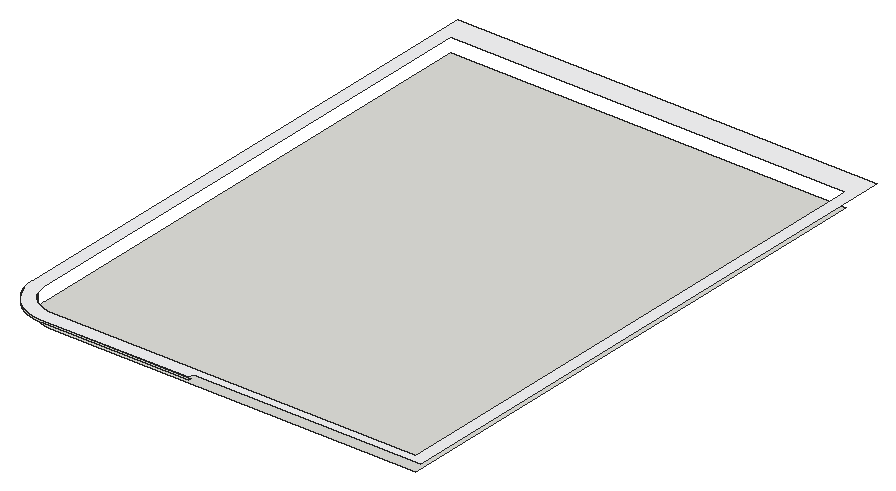
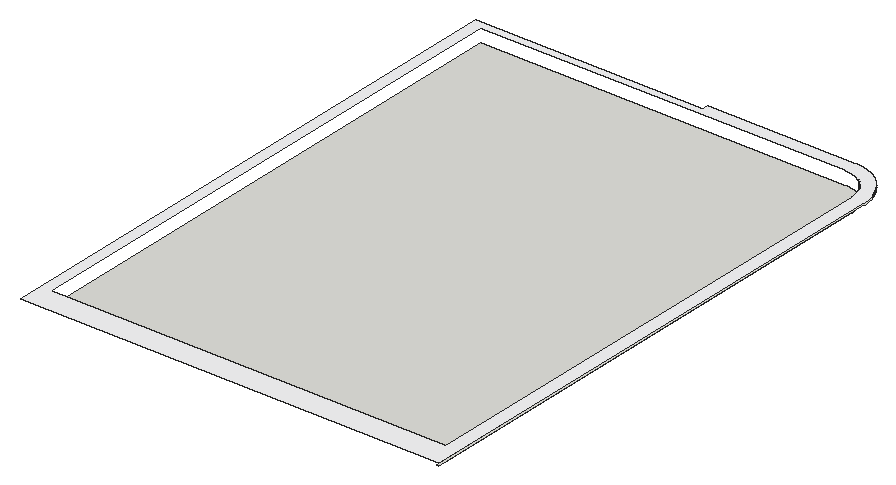
# SketchUp Ruby script. Lengths in inches.
U = 1.inch
M = Sketchup.active_model
def pt(a) = Geom::Point3d.new(a.map { |v| v * U })
def face(e, loops, mat)
  f = e.add_face(loops[0].map { |a| pt(a) })
  loops[1..].each { |l| e.add_face(l.map { |a| pt(a) }).erase! }
  f.material = f.back_material = mat if mat
  f
end
# faces: each face lists its corners as indices into pts; further lists are holes
def faces(e, pts, list, mat = nil) = list.each { |f| face(e, (f[0].is_a?(Array) ? f : [f]).map { |l| l.map { |i| pts[i] } }, mat) }
# xy, xz, yz: faces in a plane at the given z, y or x. An outline is a flat list of corners, or four numbers for a rectangle; further outlines are holes
def ring(l) = l.size == 4 ? [[l[0], l[1]], [l[2], l[1]], [l[2], l[3]], [l[0], l[3]]] : l.each_slice(2).to_a
def flat(e, list, mat, &to3) = list.each { |f| face(e, (f[0].is_a?(Array) ? f : [f]).map { |l| ring(l).map { |u, v| to3.(u, v) } }, mat) }
def xy(e, z, list, mat = nil) = flat(e, list, mat) { |x, y| [x, y, z] }
def xz(e, y, list, mat = nil) = flat(e, list, mat) { |x, z| [x, y, z] }
def yz(e, x, list, mat = nil) = flat(e, list, mat) { |y, z| [x, y, z] }
def lines(e, pts, list) = list.each { |a, b| e.add_line(pt(pts[a]), pt(pts[b])) }
# prism: a flat outline (further loops are holes) pulled along v
def prism(e, loops, v, mat = nil)
  f = face(e, loops, mat); d = Geom::Vector3d.new(v.map { |x| x * U })
  f.pushpull(f.normal.samedirection?(d) ? d.length : -d.length)
end
def box(e, o, s, mat = nil) = prism(e, [[o, [o[0] + s[0], o[1], o[2]], [o[0] + s[0], o[1] + s[1], o[2]], [o[0], o[1] + s[1], o[2]]]], [0, 0, s[2]], mat)
def at(x, y, z, deg = 0) = Geom::Transformation.translation(pt([x, y, z])) * Geom::Transformation.rotation(ORIGIN, Z_AXIS, deg.degrees)
def axes(o, x, y, z) = Geom::Transformation.new([*x, 0, *y, 0, *z, 0, *pt(o).to_a, 1])
def part(name) = M.definitions.add(name)
# library, detail: a bought-in or finely detailed component or shape, given as its bounding box
def library(name, o, s) = part(name).tap { |d| box(d.entities, o, s) }
def detail(e, o, s) = box(e.add_group.entities, o, s)
def put(e, d, t, mat = nil) = e.add_instance(d, t).tap { |i| i.material = mat if mat }
def group(e, t, mat = nil) = e.add_group.tap { |g| g.transformation = t; g.material = mat if mat }.entities
root = M.entities
M.materials.add("1122 AP 7994 PEACH ROSE").color = [254, 227, 201]
M.materials.add("[Quartz Light Grey]").color = [251, 251, 252]
xy(root,281.82,[[52.82,174,52.75,174.01,52.43,174.05,52.36,174.07,52.28,174.08,52.2,174.1,52.13,174.125,52.05,174.15,51.98,174.17,51.91,174.2,51.83,174.23,51.76,174.26,51.6875,174.29,51.62,174.33,51.55,174.36,51.41,174.44,51.35,174.48,51.28,174.53,51.22,174.57,51.15,174.62,50.97,174.77,50.86,174.88,50.8,174.93,50.6,175.17,50.55,175.24,50.51,175.3,50.46,175.37,50.42,175.43,50.34,175.57,50.31,175.64,50.27,175.71,50.18,175.92,50.15,176,50.13,176.07,50.1,176.15,50.08,176.22,50.0625,176.3,50.05,176.375,50.03,176.45,50.01,176.61,50,176.6875,49.99,176.76,49.99,176.84,49.98,176.92,49.98,177.08,49.99,177.16,49.99,177.24,50,177.3125,50.01,177.39,50.03,177.55,50.05,177.625,50.0625,177.7,50.08,177.78,50.1,177.85,50.13,177.93,50.15,178,50.18,178.08,50.27,178.29,50.31,178.36,50.34,178.43,50.42,178.57,50.46,178.63,50.51,178.7,50.55,178.76,50.6,178.83,50.8,179.07,50.86,179.12,50.97,179.23,51.15,179.38,51.22,179.43,51.28,179.47,51.35,179.52,51.41,179.56,51.55,179.64,51.62,179.67,51.6875,179.71,51.76,179.74,51.83,179.77,51.91,179.8,51.98,179.83,52.05,179.85,52.13,179.875,52.2,179.9,52.28,179.92,52.36,179.93,52.43,179.95,52.75,179.99,52.82,180,53.14,180,53.22,179.99,53.29,179.98,53.53,179.95,53.6,179.93,53.68,179.92,53.76,179.9,53.83,179.875,53.91,179.85,53.98,179.83,54.06,179.8,54.27,179.71,54.34,179.67,54.41,179.64,54.55,179.56,54.61,179.52,54.68,179.47,54.74,179.43,54.81,179.38,55.05,179.18,55.1,179.12,55.16,179.07,55.26,178.95,55.3125,178.89,55.36,178.83,55.41,178.76,55.45,178.7,55.5,178.63,55.54,178.57,55.62,178.43,55.65,178.36,55.6875,178.29,55.72,178.22,55.78,178.08,55.81,178,55.83,177.93,55.86,177.85,55.88,177.78,55.9,177.7,55.92,177.625,55.93,177.55,55.94,177.47,55.96,177.39,55.96,177.3125,55.97,177.24,55.98,177.16,55.98,176.84,55.97,176.76,55.96,176.6875,55.96,176.61,55.94,176.53,55.93,176.45,55.92,176.375,55.9,176.3,55.88,176.22,55.86,176.15,55.83,176.07,55.81,176,55.78,175.92,55.72,175.78,55.6875,175.71,55.65,175.64,55.62,175.57,55.54,175.43,55.5,175.37,55.45,175.3,55.41,175.24,55.36,175.17,55.3125,175.11,55.26,175.05,55.16,174.93,55.1,174.88,55.05,174.82,54.81,174.62,54.74,174.57,54.68,174.53,54.61,174.48,54.55,174.44,54.41,174.36,54.34,174.33,54.27,174.29,54.06,174.2,53.98,174.17,53.91,174.15,53.83,174.125,53.76,174.1,53.68,174.08,53.6,174.07,53.53,174.05,53.29,174.02,53.22,174.01,53.14,174],[164.84,174,164.76,174.01,164.6875,174.02,164.61,174.03,164.45,174.05,164.375,174.07,164.3,174.08,164.22,174.1,164.15,174.125,164.07,174.15,164,174.17,163.92,174.2,163.71,174.29,163.64,174.33,163.57,174.36,163.43,174.44,163.37,174.48,163.3,174.53,163.24,174.57,163.17,174.62,162.93,174.82,162.88,174.88,162.82,174.93,162.62,175.17,162.57,175.24,162.53,175.3,162.48,175.37,162.44,175.43,162.36,175.57,162.33,175.64,162.29,175.71,162.2,175.92,162.17,176,162.15,176.07,162.125,176.15,162.1,176.22,162.08,176.3,162.07,176.375,162.05,176.45,162.03,176.61,162.02,176.6875,162.01,176.76,162,176.84,162,177.16,162.01,177.24,162.02,177.3125,162.03,177.39,162.05,177.55,162.07,177.625,162.08,177.7,162.1,177.78,162.125,177.85,162.15,177.93,162.17,178,162.2,178.08,162.29,178.29,162.33,178.36,162.36,178.43,162.44,178.57,162.48,178.63,162.53,178.7,162.57,178.76,162.62,178.83,162.82,179.07,162.88,179.12,162.93,179.18,163.17,179.38,163.24,179.43,163.3,179.47,163.37,179.52,163.43,179.56,163.57,179.64,163.64,179.67,163.71,179.71,163.92,179.8,164,179.83,164.07,179.85,164.15,179.875,164.22,179.9,164.3,179.92,164.375,179.93,164.45,179.95,164.61,179.97,164.6875,179.98,164.76,179.99,164.84,180,165.16,180,165.24,179.99,165.3125,179.98,165.39,179.97,165.55,179.95,165.625,179.93,165.7,179.92,165.78,179.9,165.85,179.875,165.93,179.85,166,179.83,166.08,179.8,166.29,179.71,166.36,179.67,166.43,179.64,166.57,179.56,166.63,179.52,166.7,179.47,166.76,179.43,166.83,179.38,167.07,179.18,167.12,179.12,167.18,179.07,167.38,178.83,167.43,178.76,167.47,178.7,167.52,178.63,167.56,178.57,167.64,178.43,167.67,178.36,167.71,178.29,167.8,178.08,167.83,178,167.85,177.93,167.875,177.85,167.9,177.78,167.92,177.7,167.93,177.625,167.95,177.55,167.97,177.39,167.98,177.3125,167.99,177.24,168,177.16,168,176.84,167.99,176.76,167.98,176.6875,167.97,176.61,167.95,176.45,167.93,176.375,167.92,176.3,167.9,176.22,167.875,176.15,167.85,176.07,167.83,176,167.8,175.92,167.71,175.71,167.67,175.64,167.64,175.57,167.56,175.43,167.52,175.37,167.47,175.3,167.43,175.24,167.38,175.17,167.18,174.93,167.12,174.88,167.07,174.82,166.83,174.62,166.76,174.57,166.7,174.53,166.63,174.48,166.57,174.44,166.43,174.36,166.36,174.33,166.29,174.29,166.08,174.2,166,174.17,165.93,174.15,165.85,174.125,165.78,174.1,165.7,174.08,165.625,174.07,165.55,174.05,165.39,174.03,165.3125,174.02,165.24,174.01,165.16,174]],"1122 AP 7994 PEACH ROSE")
xy(root,287.82,[[44.53,162,357,162,357,624,18,624,18,188.53,18.01,188.29,18.02,188.06,18.03,187.82,18.04,187.59,18.05,187.35,18.07,187.12,18.08,186.88,18.1,186.65,18.125,186.41,18.15,186.18,18.17,185.94,18.23,185.48,18.26,185.24,18.3,185.01,18.33,184.78,18.37,184.54,18.41,184.3125,18.45,184.08,18.5,183.85,18.54,183.62,18.69,182.93,18.75,182.7,18.8,182.47,18.98,181.78,19.05,181.56,19.11,181.33,19.18,181.11,19.25,180.88,19.32,180.66,19.4,180.43,19.47,180.21,19.63,179.77,19.71,179.54,19.79,179.32,19.88,179.1,19.97,178.89,20.24,178.23,20.33,178.02,20.43,177.8,20.53,177.59,20.73,177.16,20.84,176.95,20.94,176.74,21.16,176.32,21.27,176.12,21.39,175.91,21.5,175.7,21.74,175.3,21.86,175.09,22.1,174.69,22.36,174.29,22.49,174.1,22.62,173.9,22.75,173.71,22.88,173.51,23.3,172.94,23.4375,172.75,23.58,172.5625,23.72,172.38,23.87,172.19,24.17,171.83,24.32,171.64,24.47,171.46,24.62,171.29,24.94,170.93,25.09,170.76,25.25,170.59,25.41,170.41,26.41,169.41,26.59,169.25,26.76,169.09,26.93,168.94,27.29,168.62,27.46,168.47,27.64,168.32,27.83,168.17,28.19,167.87,28.38,167.72,28.5625,167.58,28.75,167.4375,28.94,167.3,29.51,166.88,29.71,166.75,29.9,166.62,30.1,166.49,30.29,166.36,30.69,166.1,31.09,165.86,31.3,165.74,31.7,165.5,31.91,165.39,32.12,165.27,32.32,165.16,32.74,164.94,32.95,164.84,33.16,164.73,33.59,164.53,33.8,164.43,34.02,164.33,34.23,164.24,34.89,163.97,35.1,163.88,35.32,163.79,35.54,163.71,35.77,163.63,36.21,163.47,36.43,163.4,36.66,163.32,36.88,163.25,37.11,163.18,37.33,163.11,37.56,163.05,37.78,162.98,38.47,162.8,38.7,162.75,38.93,162.69,39.62,162.54,39.85,162.5,40.08,162.45,40.3125,162.41,40.54,162.37,40.78,162.33,41.01,162.3,41.24,162.26,41.48,162.23,41.94,162.17,42.18,162.15,42.41,162.125,42.65,162.1,42.88,162.08,43.12,162.07,43.35,162.05,43.59,162.04,43.82,162.03,44.06,162.02,44.29,162.01]])
xy(root,297.82,[[44.67,151,44.34,151.01,44.01,151.01,43.67,151.02,43.34,151.04,43.01,151.05,42.35,151.09,42.02,151.12,41.6875,151.14,41.36,151.17,41.03,151.21,40.7,151.24,40.37,151.28,40.04,151.33,39.71,151.37,39.38,151.42,39.06,151.47,38.73,151.52,38.4,151.58,38.08,151.64,37.42,151.76,36.78,151.9,36.45,151.97,35.49,152.21,35.16,152.29,34.84,152.38,34.53,152.47,34.21,152.56,33.57,152.76,33.26,152.86,32.94,152.96,32.32,153.18,32,153.29,31.69,153.41,31.38,153.52,31.07,153.64,30.76,153.77,30.46,153.89,30.15,154.02,29.85,154.15,29.54,154.29,29.24,154.42,28.64,154.7,28.34,154.85,28.04,154.99,27.75,155.14,27.45,155.29,27.16,155.45,26.87,155.6,26.58,155.76,26.29,155.93,26,156.09,25.71,156.26,25.15,156.6,24.86,156.77,24.3,157.13,24.03,157.3125,23.75,157.5,23.48,157.68,23.2,157.87,22.93,158.0625,22.66,158.26,22.4,158.45,22.13,158.65,21.87,158.85,21.6,159.06,21.34,159.26,21.09,159.47,20.57,159.89,20.32,160.1,19.57,160.76,19.33,160.98,19.08,161.21,18.84,161.4375,18.6,161.67,18.37,161.9,18.13,162.13,17.9,162.37,17.67,162.6,17.4375,162.84,17.21,163.08,16.98,163.33,16.76,163.57,16.1,164.32,15.89,164.57,15.47,165.09,15.26,165.34,15.06,165.6,14.85,165.87,14.65,166.13,14.45,166.4,14.26,166.66,14.0625,166.93,13.87,167.2,13.68,167.48,13.5,167.75,13.3125,168.03,13.13,168.3,12.77,168.86,12.6,169.15,12.26,169.71,12.09,170,11.93,170.29,11.76,170.58,11.6,170.87,11.45,171.16,11.29,171.45,11.14,171.75,10.99,172.04,10.85,172.34,10.7,172.64,10.42,173.24,10.29,173.54,10.15,173.85,10.02,174.15,9.89,174.46,9.77,174.76,9.64,175.07,9.52,175.38,9.41,175.69,9.29,176,9.18,176.32,8.96,176.94,8.86,177.26,8.76,177.57,8.56,178.21,8.47,178.53,8.38,178.84,8.29,179.16,8.21,179.49,7.97,180.45,7.9,180.78,7.76,181.42,7.64,182.08,7.58,182.4,7.52,182.73,7.47,183.06,7.42,183.38,7.37,183.71,7.33,184.04,7.28,184.37,7.24,184.7,7.21,185.03,7.17,185.36,7.14,185.6875,7.12,186.02,7.09,186.35,7.05,187.01,7.04,187.34,7.02,187.67,7.01,188.01,7.01,188.34,7,188.67,7,645,9,645,9,188.6875,9.01,188.37,9.01,188.06,9.02,187.74,9.03,187.43,9.05,187.12,9.07,186.8,9.11,186.18,9.14,185.86,9.2,185.24,9.23,184.92,9.35,183.99,9.4,183.68,9.44,183.37,9.49,183.06,9.55,182.75,9.6,182.44,9.72,181.82,9.79,181.52,9.85,181.21,9.92,180.9,9.99,180.6,10.07,180.29,10.15,179.99,10.23,179.68,10.39,179.08,10.48,178.78,10.57,178.47,10.67,178.17,10.76,177.875,10.86,177.58,11.06,176.98,11.17,176.6875,11.28,176.39,11.5,175.81,11.62,175.51,11.86,174.93,11.99,174.65,12.11,174.36,12.24,174.07,12.37,173.79,12.51,173.5,12.64,173.22,12.78,172.9375,12.92,172.66,13.07,172.38,13.21,172.1,13.36,171.82,13.51,171.55,13.67,171.27,13.82,171,14.3,170.19,14.47,169.92,14.64,169.66,14.81,169.39,15.15,168.87,15.69,168.09,15.875,167.84,16.0625,167.59,16.25,167.33,16.4375,167.08,16.63,166.84,16.83,166.59,17.02,166.34,17.42,165.86,17.83,165.38,18.04,165.15,18.25,164.91,18.67,164.45,18.89,164.22,19.1,163.99,19.32,163.77,19.54,163.54,19.77,163.32,19.99,163.1,20.22,162.89,20.45,162.67,20.91,162.25,21.15,162.04,21.38,161.83,21.86,161.42,22.34,161.02,22.59,160.83,22.84,160.63,23.08,160.4375,23.33,160.25,23.59,160.0625,23.84,159.875,24.09,159.69,24.87,159.15,25.39,158.81,25.66,158.64,25.92,158.47,26.19,158.3,27,157.82,27.27,157.67,27.55,157.51,27.82,157.36,28.1,157.21,28.38,157.07,28.66,156.92,28.9375,156.78,29.22,156.64,29.5,156.51,29.79,156.37,30.07,156.24,30.36,156.11,30.65,155.99,30.93,155.86,31.51,155.62,31.81,155.5,32.39,155.28,32.6875,155.17,32.98,155.06,33.58,154.86,33.875,154.76,34.17,154.67,34.47,154.57,34.78,154.48,35.08,154.39,35.68,154.23,35.99,154.15,36.29,154.07,36.6,153.99,36.9,153.92,37.21,153.85,37.52,153.79,37.82,153.72,38.44,153.6,38.75,153.55,39.06,153.49,39.37,153.44,39.68,153.4,39.99,153.35,40.92,153.23,41.24,153.2,41.86,153.14,42.18,153.11,42.8,153.07,43.12,153.05,43.43,153.03,43.74,153.02,44.06,153.01,44.37,153.01,44.6875,153,171.19,153,171.19,151]])
xy(root,299.82,[[[44.67,151,171.19,151,171.19,156,366,156,366,645,7,645,7,188.67,7.01,188.34,7.01,188.01,7.02,187.67,7.04,187.34,7.05,187.01,7.09,186.35,7.12,186.02,7.14,185.6875,7.17,185.36,7.21,185.03,7.24,184.7,7.28,184.37,7.33,184.04,7.37,183.71,7.42,183.38,7.47,183.06,7.52,182.73,7.58,182.4,7.64,182.08,7.76,181.42,7.9,180.78,7.97,180.45,8.21,179.49,8.29,179.16,8.38,178.84,8.47,178.53,8.56,178.21,8.76,177.57,8.86,177.26,8.96,176.94,9.18,176.32,9.29,176,9.41,175.69,9.52,175.38,9.64,175.07,9.77,174.76,9.89,174.46,10.02,174.15,10.15,173.85,10.29,173.54,10.42,173.24,10.7,172.64,10.85,172.34,10.99,172.04,11.14,171.75,11.29,171.45,11.45,171.16,11.6,170.87,11.76,170.58,11.93,170.29,12.09,170,12.26,169.71,12.6,169.15,12.77,168.86,13.13,168.3,13.3125,168.03,13.5,167.75,13.68,167.48,13.87,167.2,14.0625,166.93,14.26,166.66,14.45,166.4,14.65,166.13,14.85,165.87,15.06,165.6,15.26,165.34,15.47,165.09,15.89,164.57,16.1,164.32,16.76,163.57,16.98,163.33,17.21,163.08,17.4375,162.84,17.67,162.6,17.9,162.37,18.13,162.13,18.37,161.9,18.6,161.67,18.84,161.4375,19.08,161.21,19.33,160.98,19.57,160.76,20.32,160.1,20.57,159.89,21.09,159.47,21.34,159.26,21.6,159.06,21.87,158.85,22.13,158.65,22.4,158.45,22.66,158.26,22.93,158.0625,23.2,157.87,23.48,157.68,23.75,157.5,24.03,157.3125,24.3,157.13,24.86,156.77,25.15,156.6,25.71,156.26,26,156.09,26.29,155.93,26.58,155.76,26.87,155.6,27.16,155.45,27.45,155.29,27.75,155.14,28.04,154.99,28.34,154.85,28.64,154.7,29.24,154.42,29.54,154.29,29.85,154.15,30.15,154.02,30.46,153.89,30.76,153.77,31.07,153.64,31.38,153.52,31.69,153.41,32,153.29,32.32,153.18,32.94,152.96,33.26,152.86,33.57,152.76,34.21,152.56,34.53,152.47,34.84,152.38,35.16,152.29,35.49,152.21,36.45,151.97,36.78,151.9,37.42,151.76,38.08,151.64,38.4,151.58,38.73,151.52,39.06,151.47,39.38,151.42,39.71,151.37,40.04,151.33,40.37,151.28,40.7,151.24,41.03,151.21,41.36,151.17,41.6875,151.14,42.02,151.12,42.35,151.09,43.01,151.05,43.34,151.04,43.67,151.02,44.01,151.01,44.34,151.01],[44.53,162,44.29,162.01,44.06,162.02,43.82,162.03,43.59,162.04,43.35,162.05,43.12,162.07,42.88,162.08,42.65,162.1,42.41,162.125,42.18,162.15,41.94,162.17,41.48,162.23,41.24,162.26,41.01,162.3,40.78,162.33,40.54,162.37,40.3125,162.41,40.08,162.45,39.85,162.5,39.62,162.54,38.93,162.69,38.7,162.75,38.47,162.8,37.78,162.98,37.56,163.05,37.33,163.11,37.11,163.18,36.88,163.25,36.66,163.32,36.43,163.4,36.21,163.47,35.77,163.63,35.54,163.71,35.32,163.79,35.1,163.88,34.89,163.97,34.23,164.24,34.02,164.33,33.8,164.43,33.59,164.53,33.16,164.73,32.95,164.84,32.74,164.94,32.32,165.16,32.12,165.27,31.91,165.39,31.7,165.5,31.3,165.74,31.09,165.86,30.69,166.1,30.29,166.36,30.1,166.49,29.9,166.62,29.71,166.75,29.51,166.88,28.94,167.3,28.75,167.4375,28.5625,167.58,28.38,167.72,28.19,167.87,27.83,168.17,27.64,168.32,27.46,168.47,27.29,168.62,26.93,168.94,26.76,169.09,26.59,169.25,26.41,169.41,25.41,170.41,25.25,170.59,25.09,170.76,24.94,170.93,24.62,171.29,24.47,171.46,24.32,171.64,24.17,171.83,23.87,172.19,23.72,172.38,23.58,172.5625,23.4375,172.75,23.3,172.94,22.88,173.51,22.75,173.71,22.62,173.9,22.49,174.1,22.36,174.29,22.1,174.69,21.86,175.09,21.74,175.3,21.5,175.7,21.39,175.91,21.27,176.12,21.16,176.32,20.94,176.74,20.84,176.95,20.73,177.16,20.53,177.59,20.43,177.8,20.33,178.02,20.24,178.23,19.97,178.89,19.88,179.1,19.79,179.32,19.71,179.54,19.63,179.77,19.47,180.21,19.4,180.43,19.32,180.66,19.25,180.88,19.18,181.11,19.11,181.33,19.05,181.56,18.98,181.78,18.8,182.47,18.75,182.7,18.69,182.93,18.54,183.62,18.5,183.85,18.45,184.08,18.41,184.3125,18.37,184.54,18.33,184.78,18.3,185.01,18.26,185.24,18.23,185.48,18.17,185.94,18.15,186.18,18.125,186.41,18.1,186.65,18.08,186.88,18.07,187.12,18.05,187.35,18.04,187.59,18.03,187.82,18.02,188.06,18.01,188.29,18,188.53,18,624,357,624,357,162]]],"[Quartz Light Grey]")
p = [[28.94,167.3,287.82],[28.75,167.4375,287.82],[28.75,167.4375,299.82],[28.94,167.3,299.82],[28.5625,167.58,287.82],[28.5625,167.58,299.82],
  [28.38,167.72,287.82],[28.38,167.72,299.82],[28.19,167.87,287.82],[28.19,167.87,299.82],[28.01,168.02,287.82],[28.01,168.02,299.82],
  [27.83,168.17,287.82],[27.83,168.17,299.82],[27.64,168.32,287.82],[27.64,168.32,299.82],[27.46,168.47,287.82],[27.46,168.47,299.82],
  [27.29,168.62,287.82],[27.29,168.62,299.82],[27.11,168.78,287.82],[27.11,168.78,299.82],[26.93,168.94,287.82],[26.93,168.94,299.82],
  [26.76,169.09,287.82],[26.76,169.09,299.82],[26.59,169.25,287.82],[26.59,169.25,299.82],[26.41,169.41,287.82],[26.41,169.41,299.82],
  [26.24,169.58,287.82],[26.24,169.58,299.82],[26.08,169.74,287.82],[26.08,169.74,299.82],[25.91,169.91,287.82],[25.91,169.91,299.82],
  [25.74,170.08,287.82],[25.74,170.08,299.82],[25.58,170.24,287.82],[25.58,170.24,299.82],[25.41,170.41,287.82],[25.41,170.41,299.82],
  [25.25,170.59,287.82],[25.25,170.59,299.82],[25.09,170.76,287.82],[25.09,170.76,299.82],[24.94,170.93,287.82],[24.94,170.93,299.82],
  [24.78,171.11,287.82],[24.78,171.11,299.82],[24.62,171.29,287.82],[24.62,171.29,299.82],[24.47,171.46,287.82],[24.47,171.46,299.82],
  [24.32,171.64,287.82],[24.32,171.64,299.82],[24.17,171.83,287.82],[24.17,171.83,299.82],[24.02,172.01,287.82],[24.02,172.01,299.82],
  [23.87,172.19,287.82],[23.87,172.19,299.82],[23.72,172.38,287.82],[23.72,172.38,299.82],[23.58,172.5625,287.82],[23.58,172.5625,299.82],
  [23.4375,172.75,287.82],[23.4375,172.75,299.82],[23.3,172.94,287.82],[23.3,172.94,299.82],[23.16,173.13,287.82],[23.16,173.13,299.82],
  [23.02,173.32,287.82],[23.02,173.32,299.82],[22.88,173.51,287.82],[22.88,173.51,299.82],[22.75,173.71,287.82],[22.75,173.71,299.82],
  [22.62,173.9,287.82],[22.62,173.9,299.82],[22.49,174.1,287.82],[22.49,174.1,299.82],[22.36,174.29,287.82],[22.36,174.29,299.82],
  [22.23,174.49,287.82],[22.23,174.49,299.82],[22.1,174.69,287.82],[22.1,174.69,299.82],[21.98,174.89,287.82],[21.98,174.89,299.82],
  [21.86,175.09,287.82],[21.86,175.09,299.82],[21.74,175.3,287.82],[21.74,175.3,299.82],[21.62,175.5,287.82],[21.62,175.5,299.82],
  [21.5,175.7,287.82],[21.5,175.7,299.82],[21.39,175.91,287.82],[21.39,175.91,299.82],[21.27,176.12,287.82],[21.27,176.12,299.82],
  [21.16,176.32,287.82],[21.16,176.32,299.82],[21.05,176.53,287.82],[21.05,176.53,299.82],[20.94,176.74,287.82],[20.94,176.74,299.82],
  [20.84,176.95,287.82],[20.84,176.95,299.82],[20.73,177.16,287.82],[20.73,177.16,299.82],[20.63,177.375,287.82],[20.63,177.375,299.82],
  [13.5,167.75,299.82],[13.5,167.75,297.82],[13.68,167.48,297.82],[13.68,167.48,299.82],[13.3125,168.03,299.82],[13.3125,168.03,297.82],
  [13.13,168.3,299.82],[13.13,168.3,297.82],[12.95,168.58,299.82],[12.95,168.58,297.82],[12.77,168.86,299.82],[12.77,168.86,297.82],
  [12.6,169.15,299.82],[12.6,169.15,297.82],[12.43,169.43,299.82],[12.43,169.43,297.82],[12.26,169.71,299.82],[12.26,169.71,297.82],
  [12.09,170,299.82],[12.09,170,297.82],[11.93,170.29,299.82],[11.93,170.29,297.82],[11.76,170.58,299.82],[11.76,170.58,297.82],
  [11.6,170.87,299.82],[11.6,170.87,297.82],[11.45,171.16,299.82],[11.45,171.16,297.82],[11.29,171.45,299.82],[11.29,171.45,297.82],
  [11.14,171.75,299.82],[11.14,171.75,297.82],[10.99,172.04,299.82],[10.99,172.04,297.82],[10.85,172.34,299.82],[10.85,172.34,297.82],
  [10.7,172.64,299.82],[10.7,172.64,297.82],[10.56,172.94,299.82],[10.56,172.94,297.82],[10.42,173.24,299.82],[10.42,173.24,297.82],
  [10.29,173.54,299.82],[10.29,173.54,297.82],[10.15,173.85,299.82],[10.15,173.85,297.82],[10.02,174.15,299.82],[10.02,174.15,297.82],
  [9.89,174.46,299.82],[9.89,174.46,297.82],[9.77,174.76,299.82],[9.77,174.76,297.82],[9.64,175.07,299.82],[9.64,175.07,297.82],
  [9.52,175.38,299.82],[9.52,175.38,297.82],[9.41,175.69,299.82],[9.41,175.69,297.82],[9.29,176,299.82],[9.29,176,297.82],
  [9.18,176.32,299.82],[9.18,176.32,297.82],[9.07,176.63,299.82],[9.07,176.63,297.82],[8.96,176.94,299.82],[8.96,176.94,297.82],
  [8.86,177.26,299.82],[8.86,177.26,297.82],[8.76,177.57,299.82],[8.76,177.57,297.82]]
faces(root,p,[[0,1,2,3],[1,4,5,2],[4,6,7,5],[6,8,9,7],[8,10,11,9],[10,12,13,11],[12,14,15,13],[14,16,17,15],
  [16,18,19,17],[18,20,21,19],[20,22,23,21],[22,24,25,23],[24,26,27,25],[26,28,29,27],[28,30,31,29],[30,32,33,31],
  [32,34,35,33],[34,36,37,35],[36,38,39,37],[38,40,41,39],[40,42,43,41],[42,44,45,43],[44,46,47,45],[46,48,49,47],
  [48,50,51,49],[50,52,53,51],[52,54,55,53],[54,56,57,55],[56,58,59,57],[58,60,61,59],[60,62,63,61],[62,64,65,63],
  [64,66,67,65],[66,68,69,67],[68,70,71,69],[70,72,73,71],[72,74,75,73],[74,76,77,75],[76,78,79,77],[78,80,81,79],
  [80,82,83,81],[82,84,85,83],[84,86,87,85],[86,88,89,87],[88,90,91,89],[90,92,93,91],[92,94,95,93],[94,96,97,95],
  [96,98,99,97],[98,100,101,99],[100,102,103,101],[102,104,105,103],[104,106,107,105],[106,108,109,107],[108,110,111,109],[110,112,113,111]])
faces(root,p,[[114,115,116,117],[118,119,115,114],[120,121,119,118],[122,123,121,120],[124,125,123,122],[126,127,125,124],[128,129,127,126],[130,131,129,128],
  [132,133,131,130],[134,135,133,132],[136,137,135,134],[138,139,137,136],[140,141,139,138],[142,143,141,140],[144,145,143,142],[146,147,145,144],
  [148,149,147,146],[150,151,149,148],[152,153,151,150],[154,155,153,152],[156,157,155,154],[158,159,157,156],[160,161,159,158],[162,163,161,160],
  [164,165,163,162],[166,167,165,164],[168,169,167,166],[170,171,169,168],[172,173,171,170],[174,175,173,172],[176,177,175,174],[178,179,177,176],
  [180,181,179,178],[182,183,181,180]],"[Quartz Light Grey]")
